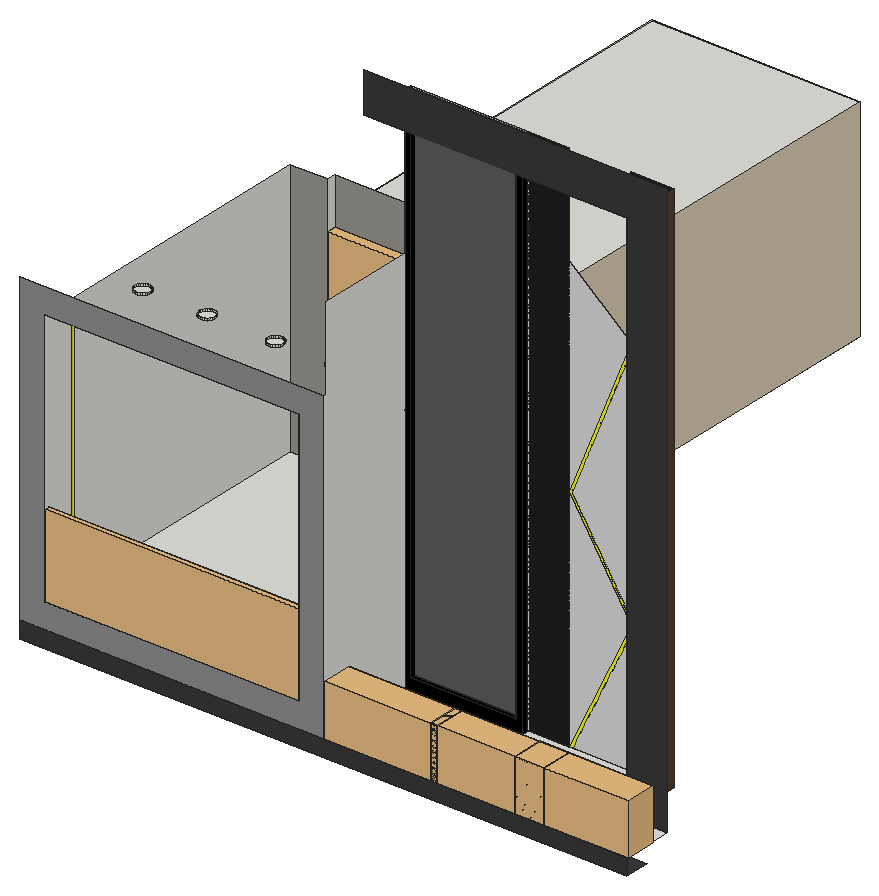
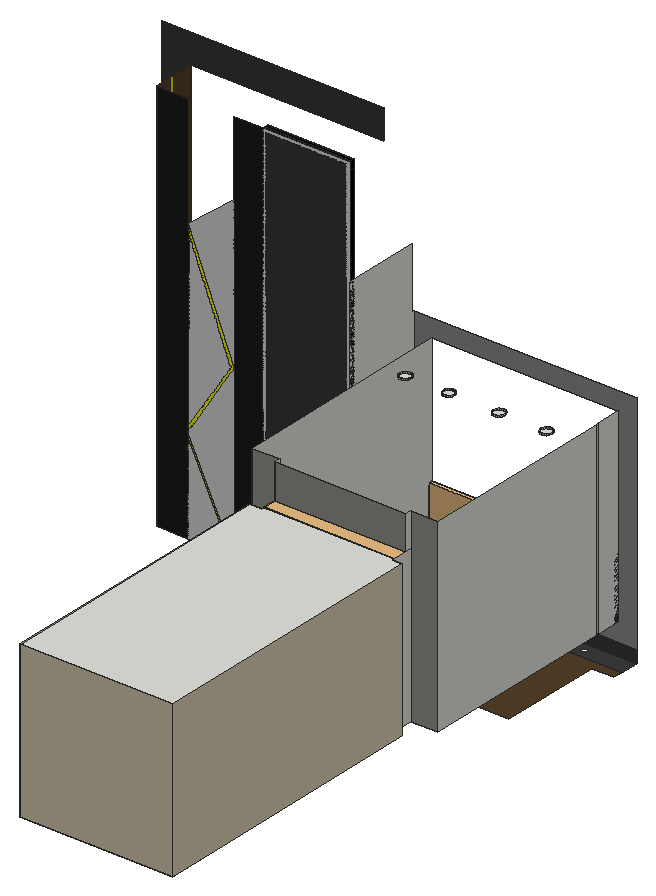
# SketchUp Ruby script. Lengths in inches.
U = 1.inch
M = Sketchup.active_model
def pt(a) = Geom::Point3d.new(a.map { |v| v * U })
def face(e, loops, mat)
  f = e.add_face(loops[0].map { |a| pt(a) })
  loops[1..].each { |l| e.add_face(l.map { |a| pt(a) }).erase! }
  f.material = f.back_material = mat if mat
  f
end
# faces: each face lists its corners as indices into pts; further lists are holes
def faces(e, pts, list, mat = nil) = list.each { |f| face(e, (f[0].is_a?(Array) ? f : [f]).map { |l| l.map { |i| pts[i] } }, mat) }
# xy, xz, yz: faces in a plane at the given z, y or x. An outline is a flat list of corners, or four numbers for a rectangle; further outlines are holes
def ring(l) = l.size == 4 ? [[l[0], l[1]], [l[2], l[1]], [l[2], l[3]], [l[0], l[3]]] : l.each_slice(2).to_a
def flat(e, list, mat, &to3) = list.each { |f| face(e, (f[0].is_a?(Array) ? f : [f]).map { |l| ring(l).map { |u, v| to3.(u, v) } }, mat) }
def xy(e, z, list, mat = nil) = flat(e, list, mat) { |x, y| [x, y, z] }
def xz(e, y, list, mat = nil) = flat(e, list, mat) { |x, z| [x, y, z] }
def yz(e, x, list, mat = nil) = flat(e, list, mat) { |y, z| [x, y, z] }
def lines(e, pts, list) = list.each { |a, b| e.add_line(pt(pts[a]), pt(pts[b])) }
# prism: a flat outline (further loops are holes) pulled along v
def prism(e, loops, v, mat = nil)
  f = face(e, loops, mat); d = Geom::Vector3d.new(v.map { |x| x * U })
  f.pushpull(f.normal.samedirection?(d) ? d.length : -d.length)
end
def box(e, o, s, mat = nil) = prism(e, [[o, [o[0] + s[0], o[1], o[2]], [o[0] + s[0], o[1] + s[1], o[2]], [o[0], o[1] + s[1], o[2]]]], [0, 0, s[2]], mat)
def at(x, y, z, deg = 0) = Geom::Transformation.translation(pt([x, y, z])) * Geom::Transformation.rotation(ORIGIN, Z_AXIS, deg.degrees)
def axes(o, x, y, z) = Geom::Transformation.new([*x, 0, *y, 0, *z, 0, *pt(o).to_a, 1])
def part(name) = M.definitions.add(name)
# library, detail: a bought-in or finely detailed component or shape, given as its bounding box
def library(name, o, s) = part(name).tap { |d| box(d.entities, o, s) }
def detail(e, o, s) = box(e.add_group.entities, o, s)
def put(e, d, t, mat = nil) = e.add_instance(d, t).tap { |i| i.material = mat if mat }
def group(e, t, mat = nil) = e.add_group.tap { |g| g.transformation = t; g.material = mat if mat }.entities
root = M.entities
M.materials.add("2").color = [128, 128, 128]
M.materials["2"].alpha = 0.5
M.materials.add("Brick Wall Grey Stone 01 200cm").color = [152, 151, 144]
M.materials.add("Generic").color = [218, 205, 180]
M.materials.add("Marble White SSS 100cm").color = [222, 222, 222]
M.materials.add("Wood Planks Pecan 33-81 150cm").color = [83, 63, 40]
M.materials.add("[0137_Black]").color = [0, 0, 0]
M.materials.add("[Color E05]").color = [239, 239, 0]
M.materials["[Color E05]"].alpha = 0.89
M.materials.add("[Color E05]1").color = [255, 255, 0]
M.materials.add("[Color M04]").color = [142, 142, 142]
M.materials.add("[Color M07]").color = [58, 58, 58]
M.materials.add("[Color M08]").color = [30, 30, 30]
c1 = library("Planted window box",[0,0,0],[56.02,15.3,25.28])
c2 = part("Window black single")
xy(c2.entities,0,[[0,0,49.21,2.52]],"[0137_Black]")
xy(c2.entities,2.71,[[2.56,0,46.5,2.52]],"[0137_Black]")
xy(c2.entities,122.09,[[2.56,0,3.15,2.52],[3.15,0,46.5,2.52]],"[0137_Black]")
xy(c2.entities,124.8,[[0,0,49.21,2.52]],"[0137_Black]")
xz(c2.entities,0,[[[0,0,49.21,124.8],[2.56,2.71,46.5,122.09]]],"[0137_Black]")
xz(c2.entities,2.52,[[2.56,2.71,46.5,122.09]],"2")
xz(c2.entities,2.52,[[[0,0,49.21,124.8],[2.56,2.71,46.5,122.09]]],"[0137_Black]")
yz(c2.entities,0,[[0,0,2.52,2.71],[0,2.71,2.52,122.09],[0,122.09,2.52,124.8]],"[0137_Black]")
yz(c2.entities,2.56,[[0,2.71,2.52,122.09]],"[0137_Black]")
yz(c2.entities,46.5,[[0,2.71,2.52,122.09]],"[0137_Black]")
yz(c2.entities,49.21,[[0,0,2.52,124.8]],"[0137_Black]")
c3 = library("My+Glass_Railing\#2",[-0.08,0,0],[124.96,2.52,40.9])
c4 = library("Group\#2",[0,0,0],[118.08,13.29,95.4])
xy(root,111.61,[[0,12.5,0,19.125,14.7,19.125,14.7,88.375,112.5,88.375,112.5,12.5]],"Wood Planks Pecan 33-81 150cm")
xy(root,111.61,[[[0,0,112.5,12.5],[29.97,4.05,30.48,4.11,30.97,4.3125,31.38,4.63,31.7,5.05,31.9,5.53,31.97,6.05,31.9,6.5625,31.7,7.05,31.38,7.46,30.97,7.78,30.48,7.98,29.97,8.05,29.45,7.98,28.97,7.78,28.55,7.46,28.23,7.05,28.03,6.5625,27.97,6.05,28.03,5.53,28.23,5.05,28.55,4.63,28.97,4.3125,29.45,4.11],[90.97,4.05,91.48,4.11,91.97,4.3125,92.38,4.63,92.7,5.05,92.9,5.53,92.97,6.05,92.9,6.5625,92.7,7.05,92.38,7.46,91.97,7.78,91.48,7.98,90.97,8.05,90.45,7.98,89.97,7.78,89.55,7.46,89.23,7.05,89.03,6.5625,88.97,6.05,89.03,5.53,89.23,5.05,89.55,4.63,89.97,4.3125,90.45,4.11]],[[112.5,0,299.0625,12.5],[237.34,4.05,237.86,4.11,238.34,4.3125,238.76,4.63,239.07,5.05,239.27,5.53,239.34,6.05,239.27,6.5625,239.07,7.05,238.76,7.46,238.34,7.78,237.86,7.98,237.34,8.05,236.82,7.98,236.34,7.78,235.93,7.46,235.61,7.05,235.41,6.5625,235.34,6.05,235.41,5.53,235.61,5.05,235.93,4.63,236.34,4.3125,236.82,4.11],[208.4,4.05,208.92,4.11,209.4,4.3125,209.82,4.63,210.14,5.05,210.34,5.53,210.4,6.05,210.34,6.5625,210.14,7.05,209.82,7.46,209.4,7.78,208.92,7.98,208.4,8.05,207.89,7.98,207.4,7.78,206.99,7.46,206.67,7.05,206.47,6.5625,206.4,6.05,206.47,5.53,206.67,5.05,206.99,4.63,207.4,4.3125,207.89,4.11],[174.28,4.05,174.8,4.11,175.28,4.3125,175.69,4.63,176.01,5.05,176.21,5.53,176.28,6.05,176.21,6.5625,176.01,7.05,175.69,7.46,175.28,7.78,174.8,7.98,174.28,8.05,173.76,7.98,173.28,7.78,172.86,7.46,172.55,7.05,172.35,6.5625,172.28,6.05,172.35,5.53,172.55,5.05,172.86,4.63,173.28,4.3125,173.76,4.11],[129.28,4.05,129.8,4.11,130.28,4.3125,130.69,4.63,131.01,5.05,131.21,5.53,131.28,6.05,131.21,6.5625,131.01,7.05,130.69,7.46,130.28,7.78,129.8,7.98,129.28,8.05,128.76,7.98,128.28,7.78,127.86,7.46,127.55,7.05,127.35,6.5625,127.28,6.05,127.35,5.53,127.55,5.05,127.86,4.63,128.28,4.3125,128.76,4.11],[267.84,4.05,268.36,4.11,268.84,4.3125,269.26,4.63,269.57,5.05,269.77,5.53,269.84,6.05,269.77,6.5625,269.57,7.05,269.26,7.46,268.84,7.78,268.36,7.98,267.84,8.05,267.32,7.98,266.84,7.78,266.43,7.46,266.11,7.05,265.91,6.5625,265.84,6.05,265.91,5.53,266.11,5.05,266.43,4.63,266.84,4.3125,267.32,4.11]]],"[Color M07]")
xy(root,120,[[149.53,0,299.0625,0,299.0625,25.125,279.23,25.125,279.23,54.0625,149.53,54.0625]])
xy(root,132.28,[[12.28,0,137.25,0,137.25,151.1875,118.84,151.1875,118.84,166.1875,126.96,166.1875,126.96,358.75,24.63,358.75,24.63,166.1875,30.69,166.1875,30.69,151.1875,12.28,151.1875]])
xy(root,235.98,[[30.69,155.4375,30.69,166.1875,24.63,166.1875,24.63,358.75,126.96,358.75,126.96,166.1875,118.84,166.1875,118.84,155.4375]])
xy(root,258.23,[[28.42,35.85,27.45,36.07,26.5625,36.52,25.83,37.19,25.29,38.03,24.99,38.98,24.94,39.97,25.15,40.94,25.61,41.83,26.28,42.5625,27.12,43.1,28.0625,43.4,29.06,43.45,30.03,43.24,30.91,42.78,31.65,42.11,32.1875,41.28,32.49,40.33,32.54,39.33,32.33,38.36,31.87,37.48,31.2,36.74,30.36,36.2,29.41,35.9],[60.17,35.85,59.2,36.07,58.3125,36.52,57.58,37.19,57.04,38.03,56.74,38.98,56.69,39.97,56.9,40.94,57.36,41.83,58.03,42.5625,58.87,43.1,59.8125,43.4,60.81,43.45,61.78,43.24,62.66,42.78,63.4,42.11,63.9375,41.28,64.24,40.33,64.29,39.33,64.08,38.36,63.62,37.48,62.95,36.74,62.11,36.2,61.16,35.9],[93.92,35.85,92.95,36.07,92.0625,36.52,91.33,37.19,90.79,38.03,90.49,38.98,90.44,39.97,90.65,40.94,91.11,41.83,91.78,42.5625,92.62,43.1,93.5625,43.4,94.56,43.45,95.53,43.24,96.41,42.78,97.15,42.11,97.6875,41.28,97.99,40.33,98.04,39.33,97.83,38.36,97.37,37.48,96.7,36.74,95.86,36.2,94.91,35.9],[123.17,35.85,122.2,36.07,121.3125,36.52,120.58,37.19,120.04,38.03,119.74,38.98,119.69,39.97,119.9,40.94,120.36,41.83,121.03,42.5625,121.87,43.1,122.8125,43.4,123.81,43.45,124.78,43.24,125.66,42.78,126.4,42.11,126.9375,41.28,127.24,40.33,127.29,39.33,127.08,38.36,126.62,37.48,125.95,36.74,125.11,36.2,124.16,35.9]])
xz(root,0,[[0,120,12.28,120,12.28,259.1,137.25,259.1,137.25,132.28,12.28,132.28,12.28,120,149.53,120,149.53,271.39,0,271.39]],"[Color M04]")
xz(root,0,[[0,111.61,299.0625,120]],"[Color M07]")
xz(root,25.125,[[279.23,120,299.0625,120,299.0625,404.5625,149.53,404.5625,149.53,384.73,279.23,384.73]],"[Color M07]")
xz(root,54.0625,[[[149.53,120,207.67,384.73],[151.65,122.12,205.55,382.61]]])
xz(root,54.0625,[[227.16,120,257.84,184.24,227.16,232.71],[229.16,120,257.84,120,257.84,180.06],[257.84,187.28,257.58,303.65,229.08,232.71],[227.16,232.71,257.84,309.1,227.16,334.74]],"Marble White SSS 100cm")
xz(root,54.0625,[[227.16,120,229.16,120,257.84,180.06,257.84,184.24],[257.84,184.24,257.84,187.28,229.08,232.71,257.58,303.65,257.84,309.1,227.16,232.71]],"[Color E05]1")
xz(root,54.0625,[[151.65,122.12,205.55,382.61]],"[Color M07]")
xz(root,54.0625,[[207.67,120,227.16,384.73],[257.84,120,279.23,120,279.23,384.73,257.84,384.73,257.84,309.1,257.58,303.65,257.84,187.28]],"[Color M08]")
xz(root,151.1875,[[12.28,132.28,30.69,259.1],[118.84,132.28,137.25,259.1]],"Brick Wall Grey Stone 01 200cm")
xz(root,155.4375,[[30.69,235.98,118.84,259.1]],"Brick Wall Grey Stone 01 200cm")
xz(root,166.1875,[[24.63,132.28,30.69,235.98],[118.84,132.28,126.96,235.98]])
xz(root,358.75,[[24.63,132.28,126.96,235.98]],"Generic")
yz(root,12.28,[[0,132.28,16.25,259.1],[18.25,132.28,151.1875,259.1]])
yz(root,12.28,[[16.25,132.28,18.25,259.1]],"[Color E05]")
yz(root,24.63,[[166.1875,132.28,358.75,235.98]],"Generic")
yz(root,30.69,[[151.1875,132.28,166.1875,235.98],[151.1875,235.98,155.4375,259.1]])
yz(root,118.84,[[151.1875,132.28,166.1875,235.98],[151.1875,235.98,155.4375,259.1]])
yz(root,126.96,[[166.1875,132.28,358.75,235.98]],"Generic")
yz(root,137.25,[[0,132.28,151.1875,259.1]])
yz(root,149.53,[[0,120,54.0625,120,54.0625,312.29,1.46,312.29,1.46,271.39,0,271.39]])
yz(root,279.23,[[25.125,120,39.59,384.73],[41.59,120,54.0625,384.73]],"Wood Planks Pecan 33-81 150cm")
yz(root,279.23,[[39.59,120,41.59,384.73]],"[Color E05]")
p = [[28.42,35.85,259.1],[27.45,36.07,259.1],[27.45,36.07,258.23],[28.42,35.85,258.23],[29.41,35.9,259.1],[29.41,35.9,258.23],
  [30.36,36.2,259.1],[30.36,36.2,258.23],[60.17,35.85,259.1],[59.2,36.07,259.1],[59.2,36.07,258.23],[60.17,35.85,258.23],
  [61.16,35.9,259.1],[61.16,35.9,258.23],[62.11,36.2,259.1],[62.11,36.2,258.23],[93.92,35.85,259.1],[92.95,36.07,259.1],
  [92.95,36.07,258.23],[93.92,35.85,258.23],[94.91,35.9,259.1],[94.91,35.9,258.23],[95.86,36.2,259.1],[95.86,36.2,258.23],
  [123.17,35.85,259.1],[122.2,36.07,259.1],[122.2,36.07,258.23],[123.17,35.85,258.23],[124.16,35.9,259.1],[124.16,35.9,258.23],
  [125.11,36.2,259.1],[125.11,36.2,258.23],[26.5625,36.52,259.1],[26.5625,36.52,258.23],[58.3125,36.52,259.1],[58.3125,36.52,258.23],
  [92.0625,36.52,259.1],[92.0625,36.52,258.23],[121.3125,36.52,259.1],[121.3125,36.52,258.23],[31.2,36.74,259.1],[31.2,36.74,258.23],
  [62.95,36.74,259.1],[62.95,36.74,258.23],[96.7,36.74,259.1],[96.7,36.74,258.23],[125.95,36.74,259.1],[125.95,36.74,258.23],
  [25.83,37.19,259.1],[25.83,37.19,258.23],[57.58,37.19,259.1],[57.58,37.19,258.23],[91.33,37.19,259.1],[91.33,37.19,258.23],
  [120.58,37.19,259.1],[120.58,37.19,258.23],[31.87,37.48,259.1],[31.87,37.48,258.23],[63.62,37.48,259.1],[63.62,37.48,258.23],
  [97.37,37.48,259.1],[97.37,37.48,258.23],[126.62,37.48,259.1],[126.62,37.48,258.23],[25.29,38.03,259.1],[25.29,38.03,258.23],
  [57.04,38.03,259.1],[57.04,38.03,258.23],[90.79,38.03,259.1],[90.79,38.03,258.23],[120.04,38.03,259.1],[120.04,38.03,258.23],
  [32.33,38.36,259.1],[32.33,38.36,258.23],[64.08,38.36,259.1],[64.08,38.36,258.23],[97.83,38.36,259.1],[97.83,38.36,258.23],
  [127.08,38.36,259.1],[127.08,38.36,258.23],[24.99,38.98,259.1],[24.99,38.98,258.23],[56.74,38.98,259.1],[56.74,38.98,258.23],
  [90.49,38.98,259.1],[90.49,38.98,258.23],[119.74,38.98,259.1],[119.74,38.98,258.23],[32.54,39.33,259.1],[32.54,39.33,258.23],
  [64.29,39.33,259.1],[64.29,39.33,258.23],[98.04,39.33,259.1],[98.04,39.33,258.23],[127.29,39.33,259.1],[127.29,39.33,258.23],
  [24.94,39.97,259.1],[24.94,39.97,258.23],[56.69,39.97,259.1],[56.69,39.97,258.23],[90.44,39.97,259.1],[90.44,39.97,258.23],
  [119.69,39.97,259.1],[119.69,39.97,258.23],[32.49,40.33,259.1],[32.49,40.33,258.23],[64.24,40.33,259.1],[64.24,40.33,258.23],
  [97.99,40.33,259.1],[97.99,40.33,258.23],[127.24,40.33,259.1],[127.24,40.33,258.23],[25.15,40.94,259.1],[25.15,40.94,258.23],
  [56.9,40.94,259.1],[56.9,40.94,258.23],[90.65,40.94,259.1],[90.65,40.94,258.23],[119.9,40.94,259.1],[119.9,40.94,258.23],
  [32.1875,41.28,259.1],[32.1875,41.28,258.23],[63.9375,41.28,259.1],[63.9375,41.28,258.23],[97.6875,41.28,259.1],[97.6875,41.28,258.23],
  [126.9375,41.28,259.1],[126.9375,41.28,258.23],[25.61,41.83,259.1],[25.61,41.83,258.23],[57.36,41.83,259.1],[57.36,41.83,258.23],
  [91.11,41.83,259.1],[91.11,41.83,258.23],[120.36,41.83,259.1],[120.36,41.83,258.23],[31.65,42.11,259.1],[31.65,42.11,258.23],
  [63.4,42.11,259.1],[63.4,42.11,258.23],[97.15,42.11,259.1],[97.15,42.11,258.23],[126.4,42.11,259.1],[126.4,42.11,258.23],
  [26.28,42.5625,259.1],[26.28,42.5625,258.23],[58.03,42.5625,259.1],[58.03,42.5625,258.23],[91.78,42.5625,259.1],[91.78,42.5625,258.23],
  [121.03,42.5625,259.1],[121.03,42.5625,258.23],[30.91,42.78,259.1],[30.91,42.78,258.23],[62.66,42.78,259.1],[62.66,42.78,258.23],
  [96.41,42.78,259.1],[96.41,42.78,258.23],[125.66,42.78,259.1],[125.66,42.78,258.23],[27.12,43.1,259.1],[27.12,43.1,258.23],
  [58.87,43.1,259.1],[58.87,43.1,258.23],[92.62,43.1,259.1],[92.62,43.1,258.23],[121.87,43.1,259.1],[121.87,43.1,258.23],
  [30.03,43.24,259.1],[30.03,43.24,258.23],[61.78,43.24,259.1],[61.78,43.24,258.23],[95.53,43.24,259.1],[95.53,43.24,258.23],
  [124.78,43.24,259.1],[124.78,43.24,258.23],[28.0625,43.4,259.1],[28.0625,43.4,258.23],[59.8125,43.4,259.1],[59.8125,43.4,258.23],
  [93.5625,43.4,259.1],[93.5625,43.4,258.23],[122.8125,43.4,259.1],[122.8125,43.4,258.23],[29.06,43.45,259.1],[29.06,43.45,258.23],
  [60.81,43.45,259.1],[60.81,43.45,258.23],[94.56,43.45,259.1],[94.56,43.45,258.23],[123.81,43.45,259.1],[123.81,43.45,258.23],
  [3944.13,1483.09,152.91],[3944.13,1483.09,154.55],[3944.13,1483.25,152.91],[3944.13,1483.25,154.55],[3911.25,1483.25,154.55],[3911.25,1483.09,154.55],
  [3911.25,1483.25,152.91],[3911.25,1483.09,152.91],[3915.96,1485.5,201.61],[3915.97,1485.5,201.61],[3942.3,1485.5,124.07],[3942.3,1485.5,124.18],
  [3913.54,1485.5,125.72],[3913.27,1485.5,125.72],[3942.92,1483.25,125.72],[3942.65,1483.25,125.72],[3943.26,1485.5,196.9],[3943.26,1485.5,197.07],
  [3914.0625,1478.88,201.63],[3914.07,1478.89,201.63]]
faces(root,p,[[0,1,2,3],[4,0,3,5],[6,4,5,7],[8,9,10,11],[12,8,11,13],[14,12,13,15],[16,17,18,19],[20,16,19,21],
  [22,20,21,23],[24,25,26,27],[28,24,27,29],[30,28,29,31],[1,32,33,2],[9,34,35,10],[17,36,37,18],[25,38,39,26],
  [40,6,7,41],[42,14,15,43],[44,22,23,45],[46,30,31,47],[32,48,49,33],[34,50,51,35],[36,52,53,37],[38,54,55,39],
  [56,40,41,57],[58,42,43,59],[60,44,45,61],[62,46,47,63],[48,64,65,49],[50,66,67,51],[52,68,69,53],[54,70,71,55],
  [72,56,57,73],[74,58,59,75],[76,60,61,77],[78,62,63,79],[64,80,81,65],[66,82,83,67],[68,84,85,69],[70,86,87,71],
  [88,72,73,89],[90,74,75,91],[92,76,77,93],[94,78,79,95],[80,96,97,81],[82,98,99,83],[84,100,101,85],[86,102,103,87],
  [104,88,89,105],[106,90,91,107],[108,92,93,109],[110,94,95,111],[96,112,113,97],[98,114,115,99],[100,116,117,101],[102,118,119,103],
  [120,104,105,121],[122,106,107,123],[124,108,109,125],[126,110,111,127],[112,128,129,113],[114,130,131,115],[116,132,133,117],[118,134,135,119],
  [136,120,121,137],[138,122,123,139],[140,124,125,141],[142,126,127,143],[128,144,145,129],[130,146,147,131],[132,148,149,133],[134,150,151,135],
  [152,136,137,153],[154,138,139,155],[156,140,141,157],[158,142,143,159],[144,160,161,145],[146,162,163,147],[148,164,165,149],[150,166,167,151],
  [168,152,153,169],[170,154,155,171],[172,156,157,173],[174,158,159,175],[160,176,177,161],[162,178,179,163],[164,180,181,165],[166,182,183,167],
  [184,168,169,185],[186,170,171,187],[188,172,173,189],[190,174,175,191],[176,184,185,177],[178,186,187,179],[180,188,189,181],[182,190,191,183]])
lines(root,p,[[192,193],[194,195],[195,193],[194,192],[196,197],[198,199],[200,201],[202,203],[204,205],[206,207],[208,209],[210,211]])
put(root,c1,at(149.53,0,120))
put(root,c1,at(202.3,0,120))
put(root,c1,at(243.99,0,120))
put(root,c2,axes([149.53,50.2,120],[1.18135,0,0],[0,1,0],[0,0,2.12119]))
put(root,c3,at(12.36,0,132.28))
put(root,c4,axes([30.69,151.1875,133.14],[0.74648,0,0],[0,1,0],[0,0,1.078]))
